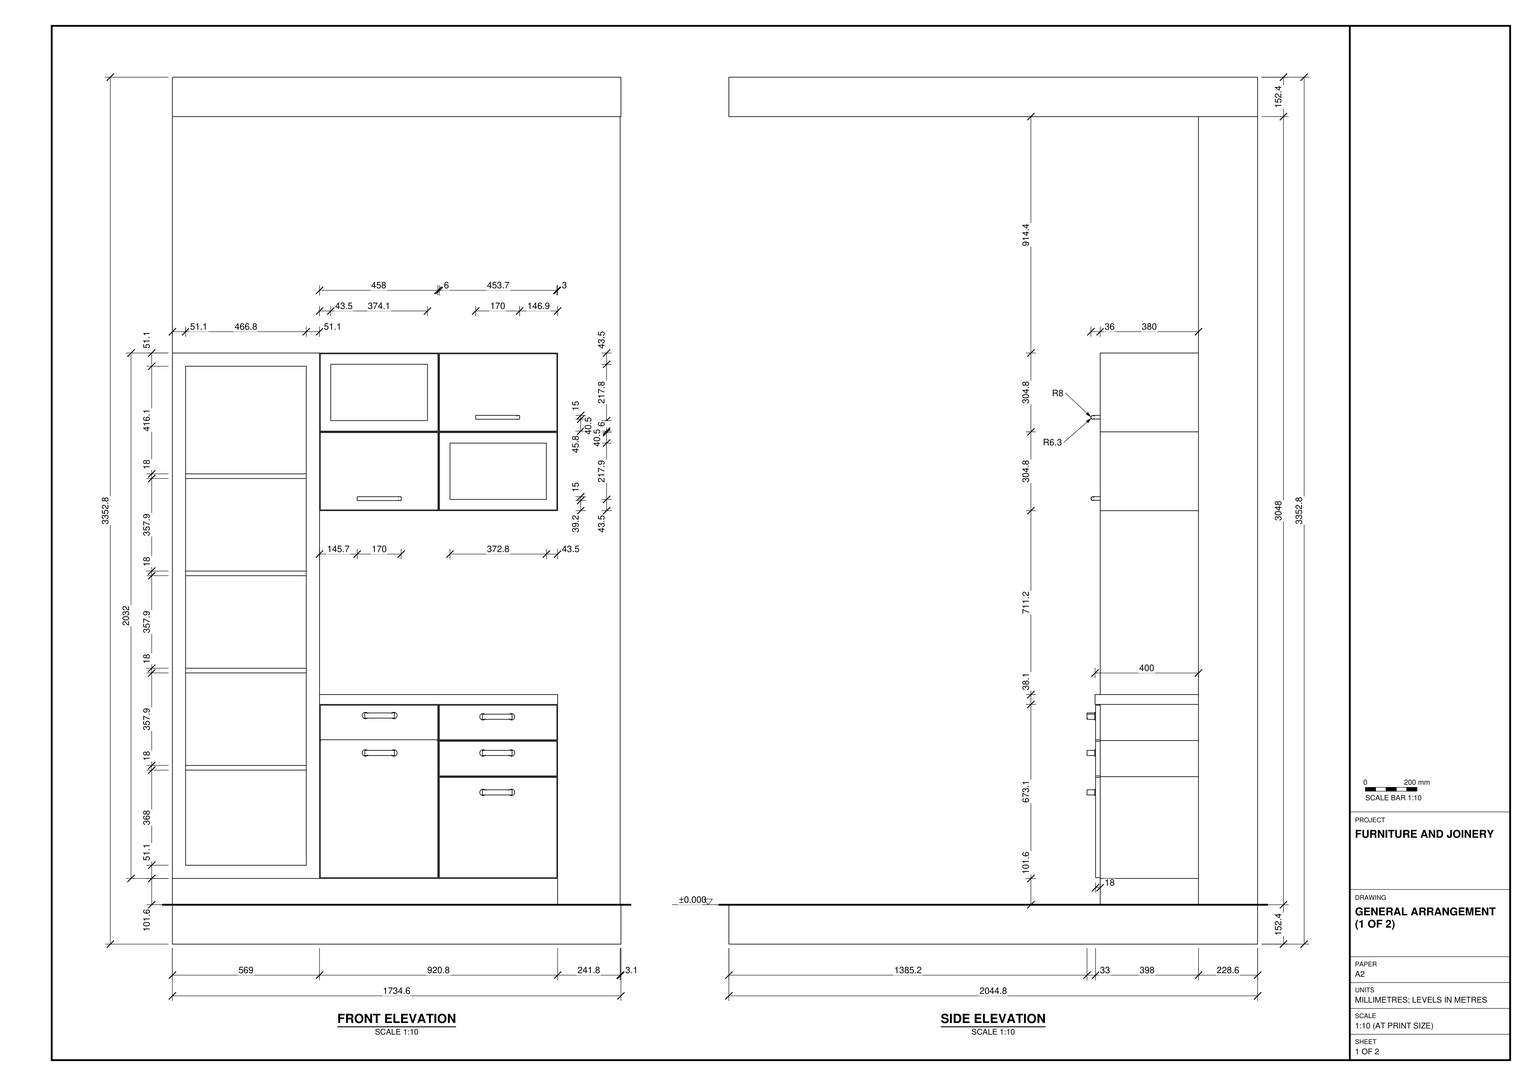
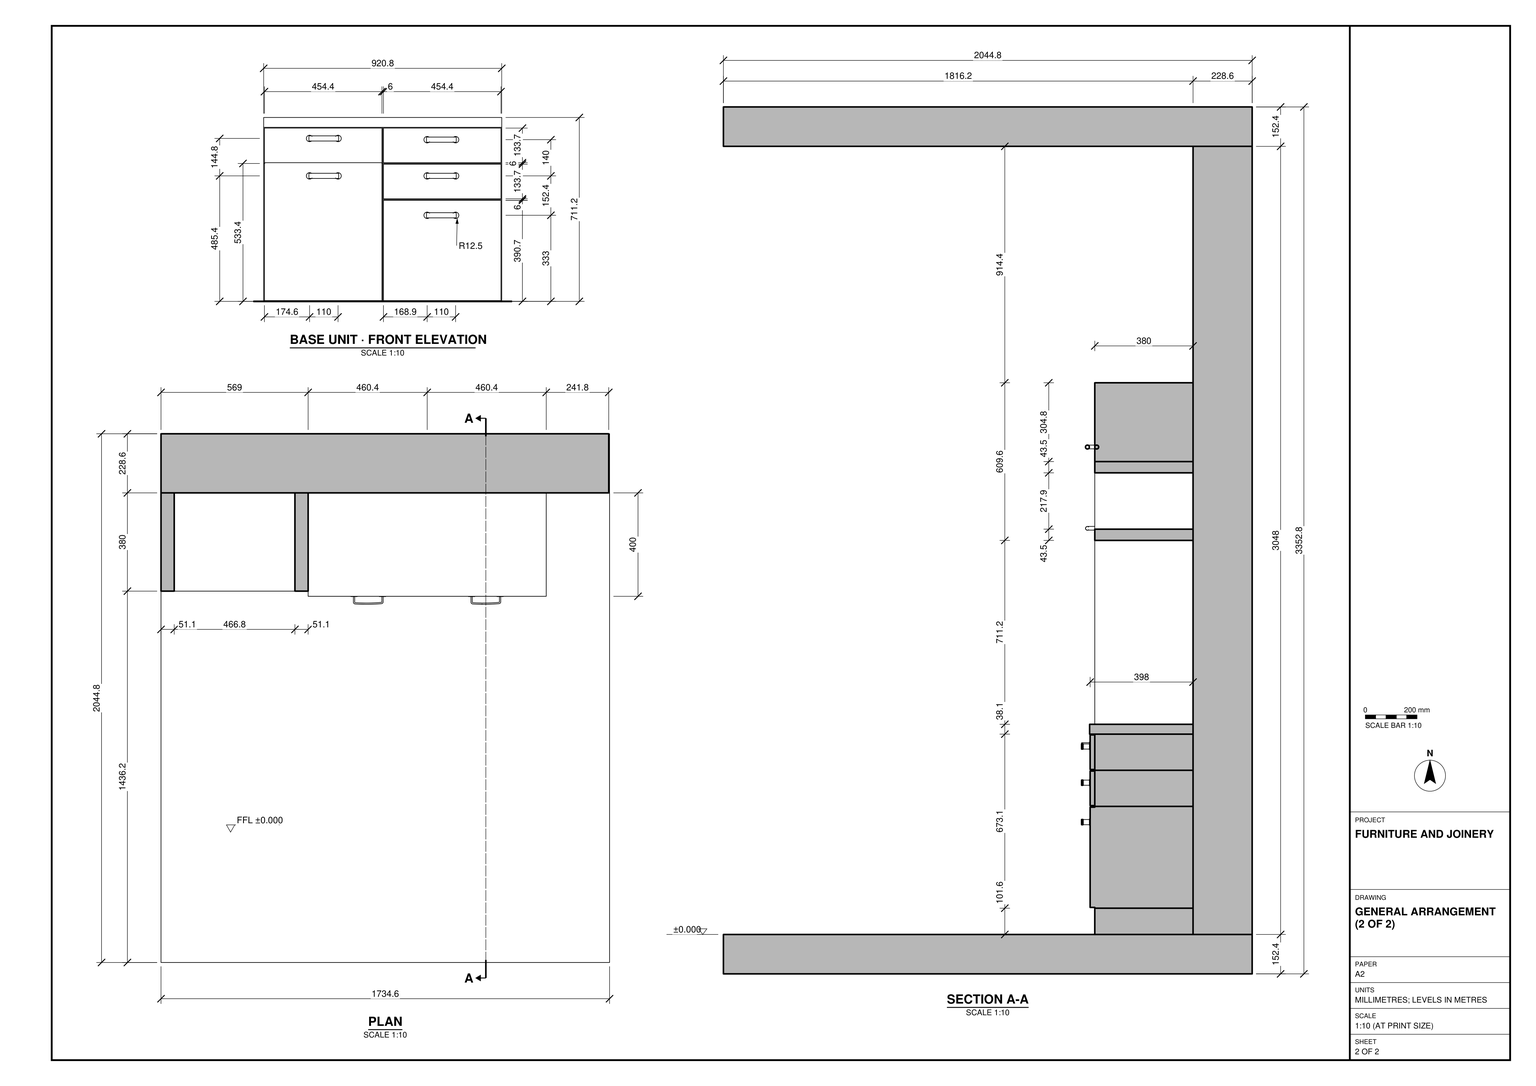
Build the storage wall in SketchUp from task_files/diagram_01.pdf. Work in millimetres. Including the shell, the model measures 1734.6 mm across the front, 2044.8 mm from front to back and 3352.8 mm high. Set the finished floor at 0 mm, the ±0.000 datum. Model the floor slab, rear wall and overhead slab at the thicknesses shown in section A-A.

Place the joinery against the rear wall, starting at the left end as seen in the front elevation. Build the tall open shelving unit with thick sides and four thinner shelves. Continue its plinth beneath the base cabinet on the right. Give the base cabinet a continuous worktop and two banks of fronts with horizontal pulls. Use the enlarged base elevation to set out the shallow fronts above the taller ones.

Above the worktop, build the wall cabinet in two tiers, with its top aligned with the tall shelving unit. Leave the upper-left and lower-right bays open and fit handled fronts to the other two bays. Preserve the clear space above the worktop and the exposed strip of rear wall to the right of the cabinets. Decor and loose items may use any suitable library components. Keep each shell element and each joinery piece in a separate group or component, and use components for repeated parts. Save one SketchUp model as output_files/storage_wall_with_open_shelving_and_cabinets.skp.

# SketchUp Ruby script. Lengths in millimetres.
U = 1.mm
M = Sketchup.active_model
def pt(a) = Geom::Point3d.new(a.map { |v| v * U })
def face(e, loops, mat)
  f = e.add_face(loops[0].map { |a| pt(a) })
  loops[1..].each { |l| e.add_face(l.map { |a| pt(a) }).erase! }
  f.material = f.back_material = mat if mat
  f
end
# faces: each face lists its corners as indices into pts; further lists are holes
def faces(e, pts, list, mat = nil) = list.each { |f| face(e, (f[0].is_a?(Array) ? f : [f]).map { |l| l.map { |i| pts[i] } }, mat) }
# xy, xz, yz: faces in a plane at the given z, y or x. An outline is a flat list of corners, or four numbers for a rectangle; further outlines are holes
def ring(l) = l.size == 4 ? [[l[0], l[1]], [l[2], l[1]], [l[2], l[3]], [l[0], l[3]]] : l.each_slice(2).to_a
def flat(e, list, mat, &to3) = list.each { |f| face(e, (f[0].is_a?(Array) ? f : [f]).map { |l| ring(l).map { |u, v| to3.(u, v) } }, mat) }
def xy(e, z, list, mat = nil) = flat(e, list, mat) { |x, y| [x, y, z] }
def xz(e, y, list, mat = nil) = flat(e, list, mat) { |x, z| [x, y, z] }
def yz(e, x, list, mat = nil) = flat(e, list, mat) { |y, z| [x, y, z] }
def lines(e, pts, list) = list.each { |a, b| e.add_line(pt(pts[a]), pt(pts[b])) }
# prism: a flat outline (further loops are holes) pulled along v
def prism(e, loops, v, mat = nil)
  f = face(e, loops, mat); d = Geom::Vector3d.new(v.map { |x| x * U })
  f.pushpull(f.normal.samedirection?(d) ? d.length : -d.length)
end
def box(e, o, s, mat = nil) = prism(e, [[o, [o[0] + s[0], o[1], o[2]], [o[0] + s[0], o[1] + s[1], o[2]], [o[0], o[1] + s[1], o[2]]]], [0, 0, s[2]], mat)
def at(x, y, z, deg = 0) = Geom::Transformation.translation(pt([x, y, z])) * Geom::Transformation.rotation(ORIGIN, Z_AXIS, deg.degrees)
def axes(o, x, y, z) = Geom::Transformation.new([*x, 0, *y, 0, *z, 0, *pt(o).to_a, 1])
def part(name) = M.definitions.add(name)
# library, detail: a bought-in or finely detailed component or shape, given as its bounding box
def library(name, o, s) = part(name).tap { |d| box(d.entities, o, s) }
def detail(e, o, s) = box(e.add_group.entities, o, s)
def put(e, d, t, mat = nil) = e.add_instance(d, t).tap { |i| i.material = mat if mat }
def group(e, t, mat = nil) = e.add_group.tap { |g| g.transformation = t; g.material = mat if mat }.entities
root = M.entities
M.materials.add("[Color E02]").color = [255, 255, 153]
M.materials.add("[Color H06]").color = [0, 204, 204]
M.materials.add("[Resin Blue]").color = [171, 210, 241]
M.materials.add("[Wood Bamboo]").color = [177, 105, 43]
c1 = library("2-POIGNEE CLC2",[-67.5,-12.5,0],[135,25,33])
c2 = library("6-POIGNEE CLC2",[-85,-7.5,0],[170,15,36])
c3 = library("10-PRODUITS CUISINE CLC2",[-119.5,-117.3,0],[240,240,120])
c4 = library("16-PRODUITS CUISINE CLC2",[-63.3,-63.3,0],[126.6,126.6,109.2])
c5 = library("23-PRODUITS CUISINE CLC2",[-125,-125,-4.7],[250,250,25])
c6 = library("15-PRODUITS CUISINE CLC2",[-49.4,-54.6,0],[100,100,140])
c7 = library("21-PRODUITS CUISINE CLC2",[-50,-50,0],[100,100,110])
c8 = library("20-PRODUITS CUISINE CLC2",[-35,-35,0],[70,70,100])
c9 = part("Group\#9")
xy(c9.entities,0,[[0,0,466.8,380]])
xy(c9.entities,18,[[0,0,466.8,380]])
xz(c9.entities,0,[[0,0,466.8,18]])
c10 = part("Group\#12")
box(c10.entities,[0,0,0],[1734.6,2044.8,152.4])
put(root,c1,axes([801.6,1418.2,1630.9],[1,0,0],[0,0,1],[0,-1,0]))
put(root,c1,axes([801.6,1418.2,1775.6],[1,0,0],[0,0,1],[0,-1,0]))
put(root,c1,axes([1256.2,1418.2,1630.9],[1,0,0],[0,0,1],[0,-1,0]))
put(root,c1,axes([1256.2,1418.2,1770.9],[1,0,0],[0,0,1],[0,-1,0]))
put(root,c1,axes([1256.2,1418.2,1478.5],[1,0,0],[0,0,1],[0,-1,0]))
put(root,c2,axes([799.7,1436.2,2614.6],[1,0,0],[0,0,1],[0,-1,0]))
put(root,c2,axes([1257.8,1472.1,2929],[1,0,0],[0,0,1],[0,-1,0]))
put(root,c2,axes([1257.8,1436.2,2929],[1,0,0],[0,0,1],[0,-1,0]))
put(root,c3,at(203.4,1436.2,2710.3))
put(root,c4,at(403.7,1499.5,2710.3))
put(root,c5,at(760.2,1599.6,1861.4))
put(root,c5,at(301.4,1561.2,2339.1))
put(root,c5,at(301.4,1561.2,2353.5))
put(root,c5,at(301.4,1561.2,2367.9))
put(root,c5,at(301.4,1561.2,2382.3))
put(root,c5,at(301.4,1561.2,2396.8))
put(root,c5,at(301.4,1561.2,1963.1))
put(root,c5,at(301.4,1561.2,1977.6))
put(root,c5,at(301.4,1561.2,2006.4))
put(root,c5,at(301.4,1561.2,1992))
put(root,c4,at(162.6,1548.3,1582.6))
put(root,c4,at(282,1548.3,1582.6))
put(root,c4,at(401.3,1548.3,1582.6))
put(root,c6,at(123.6,1576.2,1196.6))
put(root,c6,at(268.4,1576.2,1196.6))
put(root,c6,at(413.2,1576.2,1196.6))
put(root,c7,axes([669.7,1544,2916.2],[1,0,0],[0,1,0],[0,0,1.52]))
put(root,c7,axes([789.1,1544,2916.2],[1,0,0],[0,1,0],[0,0,1.52]))
put(root,c7,axes([908.5,1544,2916.2],[1,0,0],[0,1,0],[0,0,1.52]))
put(root,c8,at(1126.4,1554.1,2611.4))
put(root,c8,at(1212.8,1554.1,2611.4))
put(root,c8,at(1291.5,1554.1,2611.4))
put(root,c8,at(1372.8,1554.1,2611.4))
g1 = group(root,at(0,1436.2,1043.9))
xy(g1,0,[[0,0,1489.7,380]])
g2 = group(root,at(0,1816.2,1043.9),"[Color H06]")
xy(g2,0,[[0,0,1731.5,228.6]])
xy(g2,3048,[[0,0,1731.5,228.6]])
xz(g2,0,[[1489.7,0,1731.5,0,1731.5,3048,0,3048,0,2133.6,1489.7,2133.6,1489.7,1524,569,1524,569,812.8,1489.7,812.8]])
xz(g2,0,[[0,0,1489.7,0,1489.7,812.8,569,812.8,569,1524,1489.7,1524,1489.7,2133.6,0,2133.6]],"[Wood Bamboo]")
xz(g2,228.6,[[0,0,1731.5,3048]])
yz(g2,0,[[0,0,228.6,3048]])
yz(g2,1731.5,[[0,0,228.6,3048]])
g3 = group(root,at(0,1436.2,1043.9),"[Color E02]")
box(g3,[0,0,0],[1489.7,380,101.6])
g4 = group(root,at(569,1816.2,1818.6))
box(g4,[0,-400,0],[920.8,400,38.1])
g5 = group(root,at(569,1816.2,1145.5),"[Color E02]")
xy(g5,0,[[0,-380,460.4,0],[460.4,-380,920.8,0]])
xy(g5,3,[[3,-398,457.4,-380],[463.4,-398,917.8,-380]])
xy(g5,390.7,[[463.4,-398,917.8,-380]])
xy(g5,670.1,[[3,-398,457.4,-380]])
xy(g5,673.1,[[0,-380,460.4,0],[460.4,-380,920.8,0]])
xz(g5,-398,[[3,536.4,457.4,670.1]])
xz(g5,-398,[[3,3,457.4,536.4],[463.4,3,917.8,390.7]],"[Wood Bamboo]")
xz(g5,-380,[[[0,0,460.4,673.1],[3,3,457.4,670.1]],[[460.4,0,920.8,393.7],[463.4,3,917.8,390.7]]])
xz(g5,-380,[[460.4,393.7,920.8,673.1]],"[Wood Bamboo]")
yz(g5,0,[[-380,0,0,673.1]])
yz(g5,3,[[-398,3,-380,670.1]])
yz(g5,457.4,[[-398,3,-380,670.1]])
yz(g5,463.4,[[-398,3,-380,390.7]])
yz(g5,917.8,[[-398,3,-380,390.7]])
yz(g5,920.8,[[-380,0,0,673.1]])
g6 = group(root,at(569,1816.2,1678.9))
xy(g6,0,[[0,-380,460.4,0]])
xy(g6,3,[[3,-398,457.4,-380]])
xy(g6,136.7,[[3,-398,457.4,-380]])
xy(g6,139.7,[[0,-380,460.4,0]])
xz(g6,-380,[[[0,0,460.4,139.7],[3,3,457.4,136.7]]])
xz(g6,0,[[0,0,460.4,139.7]])
yz(g6,0,[[-380,0,0,139.7]])
yz(g6,3,[[-398,3,-380,136.7]])
yz(g6,457.4,[[-398,3,-380,136.7]])
yz(g6,460.4,[[-380,0,0,139.7]])
g7 = group(root,at(1029.3,1816.2,1678.9),"[Color E02]")
xy(g7,0,[[0,-380,460.4,0]])
xy(g7,3,[[3,-398,457.4,-380]])
xy(g7,136.7,[[3,-398,457.4,-380]])
xy(g7,139.7,[[0,-380,460.4,0]])
xz(g7,-398,[[3,3,457.4,136.7]])
xz(g7,-380,[[[0,0,460.4,139.7],[3,3,457.4,136.7]]])
xz(g7,0,[[0,0,460.4,139.7]])
yz(g7,0,[[-380,0,0,139.7]])
yz(g7,3,[[-398,3,-380,136.7]])
yz(g7,457.4,[[-398,3,-380,136.7]])
yz(g7,460.4,[[-380,0,0,139.7]])
g8 = group(root,at(1029.3,1816.2,1539.2))
xy(g8,0,[[0,-380,460.4,0]])
xy(g8,3,[[3,-398,457.4,-380]])
xy(g8,136.7,[[3,-398,457.4,-380]])
xy(g8,139.7,[[0,-380,460.4,0]])
xz(g8,-398,[[3,3,457.4,136.7]],"[Wood Bamboo]")
xz(g8,-380,[[[0,0,460.4,139.7],[3,3,457.4,136.7]]])
yz(g8,0,[[-380,0,0,139.7]])
yz(g8,3,[[-398,3,-380,136.7]])
yz(g8,457.4,[[-398,3,-380,136.7]])
g9 = group(root,at(0,1816.2,1145.5),"[Color E02]")
xy(g9,0,[[0,-380,569,0]])
xy(g9,51.1,[[51.1,-380,517.9,0]],"[Color E02]")
xy(g9,1980.9,[[51.1,-380,517.9,0]])
xy(g9,2032,[[0,-380,569,0]])
xz(g9,-380,[[[0,0,569,2032],[51.1,51.1,517.9,1980.9]]])
xz(g9,0,[[[0,0,569,2032],[51.1,51.1,517.9,1980.9]]])
yz(g9,0,[[-380,0,0,2032]])
yz(g9,51.1,[[-380,51.1,0,419.1],[-380,419.1,0,1980.9]])
yz(g9,517.9,[[-380,51.1,0,419.1],[-380,419.1,0,1980.9]])
yz(g9,569,[[-380,0,0,2032]])
put(g9,c9,at(51.1,-380,419.1),"[Color E02]")
put(g9,c9,at(51.1,-380,795))
put(g9,c9,at(51.1,-380,1170.9))
put(g9,c9,at(51.1,-380,1546.8))
g10 = group(g9,at(51.1,0,51.1),"[Wood Bamboo]")
p = [[466.8,0,1929.8],[0,0,1929.8],[0,0,0],[466.8,0,0]]
lines(g10,p,[[0,1],[1,2],[2,3],[3,0]])
g11 = group(root,at(569,1436.2,2567.9),"[Color E02]")
xy(g11,0,[[0,0,461,380],[461,0,920.8,380]])
xy(g11,43.5,[[504.5,0,877.3,380]])
xy(g11,261.3,[[504.5,0,877.3,380]])
xy(g11,304.8,[[0,0,461,380],[461,0,920.8,380]])
xy(g11,348.3,[[43.5,0,417.5,380]])
xy(g11,566.1,[[43.5,0,417.5,380]])
xy(g11,609.6,[[0,0,461,380],[461,0,920.8,380]])
xz(g11,0,[[[0,0,461,304.8],[3,3,458,301.8]],[[461,0,920.8,304.8],[464,3,917.8,301.8]],[3,3,458,301.8],[[464,3,917.8,301.8],[504.5,43.5,877.3,261.3]],[[0,304.8,461,609.6],[3,307.8,458,606.6]],
  [[461,304.8,920.8,609.6],[464,307.8,917.8,606.6]],[[3,307.8,458,606.6],[43.5,348.3,417.5,566.1]],[464,307.8,917.8,606.6]])
xz(g11,380,[[0,0,461,304.8],[[461,0,920.8,304.8],[504.5,43.5,877.3,261.3]],[461,304.8,920.8,609.6]])
yz(g11,0,[[0,0,380,304.8],[0,304.8,380,609.6]])
yz(g11,43.5,[[0,348.3,380,566.1]])
yz(g11,417.5,[[0,348.3,380,566.1]])
yz(g11,461,[[0,0,380,304.8],[0,304.8,380,609.6]])
yz(g11,504.5,[[0,43.5,380,261.3]])
yz(g11,877.3,[[0,43.5,380,261.3]])
yz(g11,920.8,[[0,0,380,304.8],[0,304.8,380,609.6]])
put(root,c10,at(0,0,891.5),"[Resin Blue]")
put(root,c10,at(0,0,4091.9))
